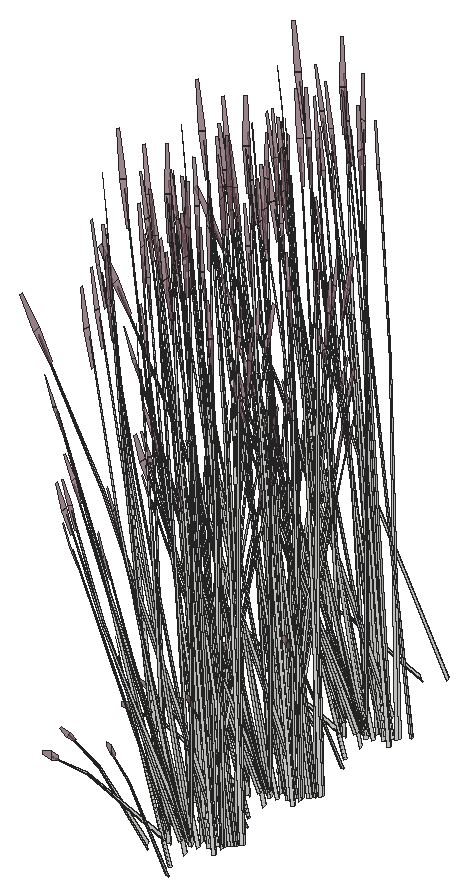
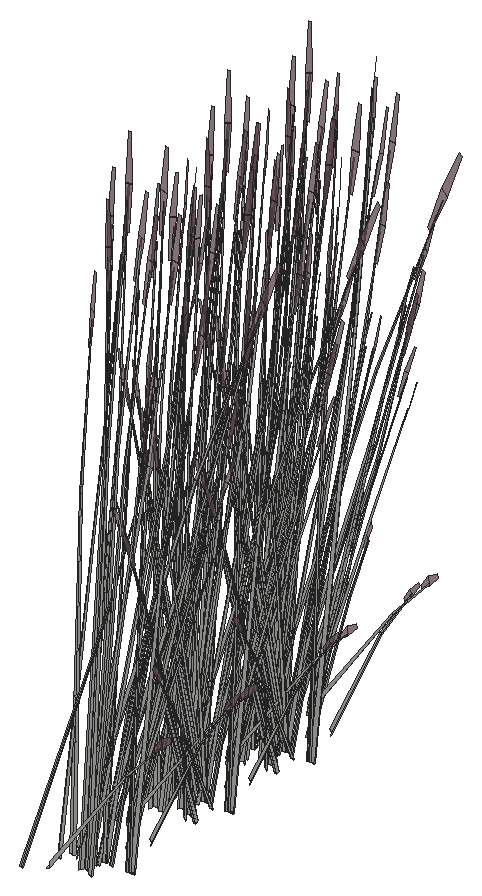
# SketchUp Ruby script. Lengths in inches.
U = 1.inch
M = Sketchup.active_model
def pt(a) = Geom::Point3d.new(a.map { |v| v * U })
def face(e, loops, mat)
  f = e.add_face(loops[0].map { |a| pt(a) })
  loops[1..].each { |l| e.add_face(l.map { |a| pt(a) }).erase! }
  f.material = f.back_material = mat if mat
  f
end
# faces: each face lists its corners as indices into pts; further lists are holes
def faces(e, pts, list, mat = nil) = list.each { |f| face(e, (f[0].is_a?(Array) ? f : [f]).map { |l| l.map { |i| pts[i] } }, mat) }
# xy, xz, yz: faces in a plane at the given z, y or x. An outline is a flat list of corners, or four numbers for a rectangle; further outlines are holes
def ring(l) = l.size == 4 ? [[l[0], l[1]], [l[2], l[1]], [l[2], l[3]], [l[0], l[3]]] : l.each_slice(2).to_a
def flat(e, list, mat, &to3) = list.each { |f| face(e, (f[0].is_a?(Array) ? f : [f]).map { |l| ring(l).map { |u, v| to3.(u, v) } }, mat) }
def xy(e, z, list, mat = nil) = flat(e, list, mat) { |x, y| [x, y, z] }
def xz(e, y, list, mat = nil) = flat(e, list, mat) { |x, z| [x, y, z] }
def yz(e, x, list, mat = nil) = flat(e, list, mat) { |y, z| [x, y, z] }
def lines(e, pts, list) = list.each { |a, b| e.add_line(pt(pts[a]), pt(pts[b])) }
# prism: a flat outline (further loops are holes) pulled along v
def prism(e, loops, v, mat = nil)
  f = face(e, loops, mat); d = Geom::Vector3d.new(v.map { |x| x * U })
  f.pushpull(f.normal.samedirection?(d) ? d.length : -d.length)
end
def box(e, o, s, mat = nil) = prism(e, [[o, [o[0] + s[0], o[1], o[2]], [o[0] + s[0], o[1] + s[1], o[2]], [o[0], o[1] + s[1], o[2]]]], [0, 0, s[2]], mat)
def at(x, y, z, deg = 0) = Geom::Transformation.translation(pt([x, y, z])) * Geom::Transformation.rotation(ORIGIN, Z_AXIS, deg.degrees)
def axes(o, x, y, z) = Geom::Transformation.new([*x, 0, *y, 0, *z, 0, *pt(o).to_a, 1])
def part(name) = M.definitions.add(name)
# library, detail: a bought-in or finely detailed component or shape, given as its bounding box
def library(name, o, s) = part(name).tap { |d| box(d.entities, o, s) }
def detail(e, o, s) = box(e.add_group.entities, o, s)
def put(e, d, t, mat = nil) = e.add_instance(d, t).tap { |i| i.material = mat if mat }
def group(e, t, mat = nil) = e.add_group.tap { |g| g.transformation = t; g.material = mat if mat }.entities
root = M.entities
M.materials.add("LightPink_Translucent").color = [144, 107, 117]
M.materials["LightPink_Translucent"].alpha = 0.75
c1 = part("blade")
p = [[2.15,0.21,22],[0,0.17,0],[0.09,0.45,0],[2.18,0.31,22],[2.29,0.31,22],[0.38,0.45,0],
  [2.48,0.24,33],[2.49,0.24,33],[2.48,0.22,33]]
faces(c1.entities,p,[[0,1,2,3],[4,5,2,3],[6,3,4,7],[8,0,3,6]])
c2 = part("seeds")
p = [[0.3,-0.1,1.38],[-0.01,-0.03,1.59],[-0.01,-0.03,0.03],[0.14,-0.07,-0.07],[0.29,-0.03,3],[0.15,0.01,3.11]]
faces(c2.entities,p,[[0,1,2,3],[1,0,4,5]],"LightPink_Translucent")
c3 = part("blade with seeds")
put(c3.entities,c1,at(0,0,0))
put(c3.entities,c2,axes([2.4,0.25,30.99],[1.5799,-0.05474,1.17369],[-0.12525,1.92788,0.29478],[-0.07173,-0.02425,1.56792]))
put(root,c3,axes([343.98,57.74,7.01],[-0.13683,-0.09148,1.74944],[-0.91315,0.058,-0.27667],[-0.14574,-0.2188,0.14031]))
put(root,c3,axes([344.94,59.28,7.27],[-0.42698,-0.53052,-0.71045],[0.87893,-0.29566,0.08574],[-0.09984,-0.25633,1.00501]))
put(root,c3,axes([344.2,58.1,3.79],[-0.15005,0.02351,1.76342],[-0.82981,-0.26461,-0.26939],[0.01392,-0.22072,0.30037]))
put(root,c3,axes([345.02,58.83,6.82],[0.2697,-0.50175,-0.35414],[0.78684,0.14635,0.4572],[-0.07215,-0.20201,0.87481]))
put(root,c3,axes([344.62,59.17,6.97],[-0.87941,-0.16356,-0.51099],[0.30143,-0.56078,-0.3958],[-0.08064,-0.22578,0.97773]))
put(root,c3,axes([342.87,58.82,7.39],[0.99656,-0.1677,0.53763],[0.17295,0.65785,0.4433],[-0.23438,-0.19388,1.11249]))
put(root,c3,axes([345.37,59.15,7.33],[-0.87543,0.30377,-0.1216],[-0.4302,-0.53915,-0.67495],[-0.1155,-0.2272,1.02557]))
put(root,c3,axes([341.89,58.23,5.06],[0.46666,0.22709,1.1486],[-0.67962,0.13651,0.84392],[-0.14541,-0.17452,0.25299]))
put(root,c3,axes([343.09,58.97,7.02],[0.4066,-0.41448,0.0643],[0.57901,0.24131,0.50621],[-0.18719,-0.13288,0.77189]))
put(root,c3,axes([342.97,61.27,4.39],[-0.36739,-0.66907,-0.69835],[1.05831,-0.24096,-0.18329],[-0.04061,-0.22656,1.54149]))
put(root,c3,axes([345.11,59.36,7.34],[-0.2697,0.50175,0.35414],[-0.78684,-0.14635,-0.4572],[-0.07215,-0.20201,0.87481]))
put(root,c3,axes([344.05,58.5625,4.42],[-0.61821,0.37431,-0.03893],[-0.56645,-0.40995,-0.17649],[-0.03988,-0.11616,0.58215]))
put(root,c3,axes([344.84,63,5.62],[0.77308,0.2631,1.51261],[-0.75736,0.56681,0.59816],[-0.33924,-0.33594,1.26806]))
put(root,c3,axes([343.22,59.44,7.34],[0.13817,0.52554,0.35414],[-0.78985,0.13877,-0.4572],[-0.21215,-0.1506,0.87481]))
put(root,c3,axes([340.8,61.18,4.3125],[0,-0.65246,-0.49651],[1.00089,0,0],[0,-0.1486,1.57504]))
put(root,c3,axes([341.23,61.19,4.32],[0.62448,-0.40708,-0.30978],[0.62448,0.40708,0.30978],[0,-0.13112,1.38974]))
put(root,c3,axes([343.42,61.94,4.96],[-1.00749,-0.31132,-0.29095],[0.48511,-0.65709,-0.50002],[-0.03166,-0.16133,1.59708]))
put(root,c3,axes([341.42,61.48,4.625],[-0.83213,0.54855,0.30756],[-0.83263,-0.54278,-0.36492],[-0.02906,-0.15578,1.64885]))
put(root,c3,axes([343.67,62.625,4.73],[0.23711,-0.77313,-0.23429],[1.12425,0.13477,0.51271],[-0.19645,-0.10677,1.5644]))
put(root,c3,axes([341.23,61.79,4.77],[0,0.65246,0.49651],[-1.00089,0,0],[0,-0.1486,1.57504]))
put(root,c3,axes([343.59,62.3125,4.5],[-0.53742,-0.54764,-0.44739],[0.81403,-0.38564,0.21531],[-0.17391,-0.06776,1.43643]))
put(root,c3,axes([343.7,61.54,4.65],[0.38895,0.72959,0.45755],[-1.11135,0.2537,0.17955],[0.01358,-0.13406,1.58856]))
put(root,c3,axes([343.51,62.11,5.01],[-0.43405,0.58792,0.44739],[-0.90188,-0.28295,-0.21531],[0,-0.13553,1.43643]))
put(root,c3,axes([345.38,62.1875,4.59],[-0.83213,-0.56158,-0.06131],[0.83263,-0.56193,0],[-0.02906,-0.01961,1.75571]))
put(root,c3,axes([343.8,62.25,4.65],[1.13071,0.13747,0.45755],[-0.23011,0.77639,0.17955],[-0.16524,-0.07497,1.58856]))
put(root,c3,axes([343.19,63.49,4.77],[0.96132,-0.17317,0.17642],[0.23737,0.64447,0.35086],[-0.08574,-0.0939,1.60407]))
put(root,c3,axes([344.08,62.81,4.91],[-0.17258,0.58229,0.1448],[-0.84319,-0.10108,-0.41347],[-0.15345,-0.05979,1.26744]))
put(root,c3,axes([346.05,63.53,4.77],[0.25843,-0.64844,0.17642],[0.9457,0.1835,0.35086],[-0.16336,0.00316,1.60407]))
put(root,c3,axes([344.43,63.6,4.49],[-0.90188,-0.29293,0],[0.43405,-0.60866,0],[0,0,1.62707]))
put(root,c3,axes([345.18,62.82,4.76],[-0.87356,-0.52515,-0.25192],[0.73507,-0.5897,0.5513],[-0.23523,0.06143,1.68216]))
put(root,c3,axes([342.88,63.82,4.77],[0.83726,0.32623,0.49651],[-0.50045,0.58498,0],[-0.19069,-0.0743,1.57504]))
put(root,c3,axes([343.98,67.5625,7.01],[-0.13683,-0.09148,1.74944],[-0.91315,0.058,-0.27667],[-0.14574,-0.2188,0.14031]))
put(root,c3,axes([344.94,69.11,7.27],[-0.42698,-0.53052,-0.71045],[0.87893,-0.29566,0.08574],[-0.09984,-0.25633,1.00501]))
put(root,c3,axes([345.6,62.38,5.01],[0.97146,-0.04028,0.44739],[0.08785,0.66859,-0.21531],[-0.17391,0.06776,1.43643]))
put(root,c3,axes([344.74,62.71,4.5],[-0.97146,0.04028,-0.44739],[-0.08785,-0.66859,0.21531],[-0.17391,0.06776,1.43643]))
put(root,c3,axes([344.2,67.93,3.79],[-0.15005,0.02351,1.76342],[-0.82981,-0.26461,-0.26939],[0.01392,-0.22072,0.30037]))
put(root,c3,axes([345.02,68.66,6.82],[0.2697,-0.50175,-0.35414],[0.78684,0.14635,0.4572],[-0.07215,-0.20201,0.87481]))
put(root,c3,axes([345.8125,64.26,4.49],[-0.55235,-0.65609,-0.05142],[0.93577,-0.36461,0.51607],[-0.23059,0.06247,1.6363]))
put(root,c3,axes([345.62,62.67,4.91],[0.66093,0.39201,0.1448],[-0.5513,0.44227,-0.41347],[-0.15345,0.05979,1.26744]))
put(root,c3,axes([344.62,69,6.97],[-0.87941,-0.16356,-0.51099],[0.30143,-0.56078,-0.3958],[-0.08064,-0.22578,0.97773]))
put(root,c3,axes([346.32,63.88,4.77],[0.83726,-0.32623,0.49651],[0.50045,0.58498,0],[-0.19069,0.0743,1.57504]))
put(root,c3,axes([345.5625,64.17,4.32],[-0.83462,-0.16144,-0.30978],[0.21015,-0.56852,0.30978],[-0.16826,0.06556,1.38974]))
put(root,c3,axes([342.87,68.65,7.39],[0.99656,-0.1677,0.53763],[0.17295,0.65785,0.4433],[-0.23438,-0.19388,1.11249]))
put(root,c3,axes([345.37,68.97,7.33],[-0.87543,0.30377,-0.1216],[-0.4302,-0.53915,-0.67495],[-0.1155,-0.2272,1.02557]))
put(root,c3,axes([341.89,68.05,5.06],[0.46666,0.22709,1.1486],[-0.67962,0.13651,0.84392],[-0.14541,-0.17452,0.25299]))
put(root,c3,axes([345.42,62.52,4.96],[0.10425,0.7445,-0.29095],[-1.08575,0.04502,-0.50002],[-0.19119,0.09917,1.59708]))
put(root,c3,axes([343.09,68.79,7.02],[0.4066,-0.41448,0.0643],[0.57901,0.24131,0.50621],[-0.18719,-0.13288,0.77189]))
put(root,c3,axes([344.77,63.09,4.35],[-0.60257,0.49041,-0.62353],[-0.74854,-0.44469,-0.16365],[-0.24146,0.12234,1.37633]))
put(root,c3,axes([342.97,71.1,4.39],[-0.36739,-0.66907,-0.69835],[1.05831,-0.24096,-0.18329],[-0.04061,-0.22656,1.54149]))
put(root,c3,axes([345.84,63.92,4.625],[1.11998,0.21207,0.30756],[-0.2802,0.75803,-0.36492],[-0.18537,0.09487,1.64885]))
put(root,c3,axes([345.76,64.43,4.3125],[-0.83726,0.32623,-0.49651],[-0.50045,-0.58498,0],[-0.19069,0.0743,1.57504]))
put(root,c3,axes([345.11,69.1875,7.34],[-0.2697,0.50175,0.35414],[-0.78684,-0.14635,-0.4572],[-0.07215,-0.20201,0.87481]))
put(root,c3,axes([344.05,68.39,4.42],[-0.61821,0.37431,-0.03893],[-0.56645,-0.40995,-0.17649],[-0.03988,-0.11616,0.58215]))
put(root,c3,axes([341.98,63.63,7.34],[0.60531,-0.34352,0.35414],[0.573,0.39225,-0.4572],[-0.08718,0.19929,0.87481]))
put(root,c3,axes([346.52,64.33,4.67],[0.55932,0.6538,0],[-0.93577,0.36461,-0.51607],[-0.21313,0.08304,1.63711]))
put(root,c3,axes([346.04,61.74,5.13],[-0.02444,-0.61432,1.41272],[1.10603,0.15924,0.59816],[-0.26159,0.33615,1.3335]))
put(root,c3,axes([344.84,72.83,5.62],[0.77308,0.2631,1.51261],[-0.75736,0.56681,0.59816],[-0.33924,-0.33594,1.26806]))
put(root,c3,axes([343.22,69.27,7.34],[0.13817,0.52554,0.35414],[-0.78985,0.13877,-0.4572],[-0.21215,-0.1506,0.87481]))
put(root,c3,axes([340.8,71.01,4.3125],[0,-0.65246,-0.49651],[1.00089,0,0],[0,-0.1486,1.57504]))
put(root,c3,axes([343.4375,64.65,7.02],[-0.6592,0.22175,0.0643],[-0.32265,-0.40436,0.50621],[0.06366,0.17825,0.77189]))
put(root,c3,axes([341.23,71.02,4.32],[0.62448,-0.40708,-0.30978],[0.62448,0.40708,0.30978],[0,-0.13112,1.38974]))
put(root,c3,axes([341.67,64.12,6.82],[-0.60531,0.34352,-0.35414],[-0.573,-0.39225,0.4572],[-0.08718,0.19929,0.87481]))
put(root,c3,axes([341.6,63.73,7.69],[0.98321,0.03233,-0.13498],[-0.02687,0.61208,-0.74919],[-0.0683,0.23574,1.13838]))
put(root,c3,axes([343.67,64.61,7.36],[-0.88151,-0.17057,0.53283],[0.30143,-0.56078,0.43934],[0.05297,0.22053,1.10256]))
put(root,c3,axes([343.42,71.76,4.96],[-1.00749,-0.31132,-0.29095],[0.48511,-0.65709,-0.50002],[-0.03166,-0.16133,1.59708]))
put(root,c3,axes([342.05,65.46,5.06],[-0.02315,-0.38796,1.1486],[0.57853,0.27671,0.84392],[-0.11378,0.18492,0.25299]))
put(root,c3,axes([342.27,63.96,7.3],[0.64041,0.4384,-0.5672],[-0.67652,0.38394,-0.43934],[-0.09744,0.22274,1.08528]))
put(root,c3,axes([341.57,64.62,5.12],[0.8127,-0.11554,0.06507],[0.18684,0.46549,-0.86304],[-0.05152,0.23564,0.7736]))
put(root,c3,axes([341.42,71.31,4.625],[-0.83213,0.54855,0.30756],[-0.83263,-0.54278,-0.36492],[-0.02906,-0.15578,1.64885]))
put(root,c3,axes([342.07,63.76,7.63],[-0.02328,0.60353,-0.7886],[-0.98022,-0.04053,0.09517],[-0.10344,0.25568,1.11556]))
put(root,c3,axes([339.51,65.34,7],[0.10149,-0.03939,1.77383],[0.83886,0.26202,-0.16761],[-0.01971,0.21816,0.31391]))
put(root,c3,axes([343.67,72.45,4.73],[0.23711,-0.77313,-0.23429],[1.12425,0.13477,0.51271],[-0.19645,-0.10677,1.5644]))
put(root,c3,axes([343,63.33,6.17],[-0.0219,-0.25042,1.71376],[0.94901,0.16613,0.13857],[-0.0587,0.35688,0.73262]))
put(root,c3,axes([341.23,71.61,4.77],[0,0.65246,0.49651],[-1.00089,0,0],[0,-0.1486,1.57504]))
put(root,c3,axes([343.59,72.14,4.5],[-0.53742,-0.54764,-0.44739],[0.81403,-0.38564,0.21531],[-0.17391,-0.06776,1.43643]))
put(root,c3,axes([343.7,71.37,4.65],[0.38895,0.72959,0.45755],[-1.11135,0.2537,0.17955],[0.01358,-0.13406,1.58856]))
put(root,c3,axes([343.51,71.94,5.01],[-0.43405,0.58792,0.44739],[-0.90188,-0.28295,-0.21531],[0,-0.13553,1.43643]))
put(root,c3,axes([341.74,64.61,5.66],[0.01966,-0.33682,1.54345],[0.88405,0.17791,0.21329],[-0.0766,0.35897,0.72882]))
put(root,c3,axes([345.38,72.01,4.59],[-0.83213,-0.56158,-0.06131],[0.83263,-0.56193,0],[-0.02906,-0.01961,1.75571]))
put(root,c3,axes([343.8,72.08,4.65],[1.13071,0.13747,0.45755],[-0.23011,0.77639,0.17955],[-0.16524,-0.07497,1.58856]))
put(root,c3,axes([343.19,73.32,4.77],[0.96132,-0.17317,0.17642],[0.23737,0.64447,0.35086],[-0.08574,-0.0939,1.60407]))
put(root,c3,axes([344.08,72.64,4.91],[-0.17258,0.58229,0.1448],[-0.84319,-0.10108,-0.41347],[-0.15345,-0.05979,1.26744]))
put(root,c3,axes([346.05,73.36,4.77],[0.25843,-0.64844,0.17642],[0.9457,0.1835,0.35086],[-0.16336,0.00316,1.60407]))
put(root,c3,axes([344.43,73.42,4.49],[-0.90188,-0.29293,0],[0.43405,-0.60866,0],[0,0,1.62707]))
put(root,c3,axes([345.18,72.64,4.76],[-0.87356,-0.52515,-0.25192],[0.73507,-0.5897,0.5513],[-0.23523,0.06143,1.68216]))
put(root,c3,axes([342.88,73.65,4.77],[0.83726,0.32623,0.49651],[-0.50045,0.58498,0],[-0.19069,-0.0743,1.57504]))
put(root,c3,axes([345.6,72.21,5.01],[0.97146,-0.04028,0.44739],[0.08785,0.66859,-0.21531],[-0.17391,0.06776,1.43643]))
put(root,c3,axes([344.74,72.53,4.5],[-0.97146,0.04028,-0.44739],[-0.08785,-0.66859,0.21531],[-0.17391,0.06776,1.43643]))
put(root,c3,axes([345.8125,74.08,4.49],[-0.55235,-0.65609,-0.05142],[0.93577,-0.36461,0.51607],[-0.23059,0.06247,1.6363]))
put(root,c3,axes([345.62,72.5,4.91],[0.66093,0.39201,0.1448],[-0.5513,0.44227,-0.41347],[-0.15345,0.05979,1.26744]))
put(root,c3,axes([346.32,73.7,4.77],[0.83726,-0.32623,0.49651],[0.50045,0.58498,0],[-0.19069,0.0743,1.57504]))
put(root,c3,axes([345.5625,74,4.32],[-0.83462,-0.16144,-0.30978],[0.21015,-0.56852,0.30978],[-0.16826,0.06556,1.38974]))
put(root,c3,axes([345.42,72.35,4.96],[0.10425,0.7445,-0.29095],[-1.08575,0.04502,-0.50002],[-0.19119,0.09917,1.59708]))
put(root,c3,axes([343.98,79.5625,7.01],[-0.13683,-0.09148,1.74944],[-0.91315,0.058,-0.27667],[-0.14574,-0.2188,0.14031]))
put(root,c3,axes([344.94,81.11,7.27],[-0.42698,-0.53052,-0.71045],[0.87893,-0.29566,0.08574],[-0.09984,-0.25633,1.00501]))
put(root,c3,axes([344.77,72.92,4.35],[-0.60257,0.49041,-0.62353],[-0.74854,-0.44469,-0.16365],[-0.24146,0.12234,1.37633]))
put(root,c3,axes([344.2,79.93,3.79],[-0.15005,0.02351,1.76342],[-0.82981,-0.26461,-0.26939],[0.01392,-0.22072,0.30037]))
put(root,c3,axes([345.84,73.75,4.625],[1.11998,0.21207,0.30756],[-0.2802,0.75803,-0.36492],[-0.18537,0.09487,1.64885]))
put(root,c3,axes([345.76,74.26,4.3125],[-0.83726,0.32623,-0.49651],[-0.50045,-0.58498,0],[-0.19069,0.0743,1.57504]))
put(root,c3,axes([345.02,80.66,6.82],[0.2697,-0.50175,-0.35414],[0.78684,0.14635,0.4572],[-0.07215,-0.20201,0.87481]))
put(root,c3,axes([344.62,81,6.97],[-0.87941,-0.16356,-0.51099],[0.30143,-0.56078,-0.3958],[-0.08064,-0.22578,0.97773]))
put(root,c3,axes([341.98,73.46,7.34],[0.60531,-0.34352,0.35414],[0.573,0.39225,-0.4572],[-0.08718,0.19929,0.87481]))
put(root,c3,axes([346.52,74.16,4.67],[0.55932,0.6538,0],[-0.93577,0.36461,-0.51607],[-0.21313,0.08304,1.63711]))
put(root,c3,axes([346.04,71.57,5.13],[-0.02444,-0.61432,1.41272],[1.10603,0.15924,0.59816],[-0.26159,0.33615,1.3335]))
put(root,c3,axes([342.87,80.65,7.39],[0.99656,-0.1677,0.53763],[0.17295,0.65785,0.4433],[-0.23438,-0.19388,1.11249]))
put(root,c3,axes([345.37,80.97,7.33],[-0.87543,0.30377,-0.1216],[-0.4302,-0.53915,-0.67495],[-0.1155,-0.2272,1.02557]))
put(root,c3,axes([341.89,80.05,5.06],[0.46666,0.22709,1.1486],[-0.67962,0.13651,0.84392],[-0.14541,-0.17452,0.25299]))
put(root,c3,axes([343.09,80.79,7.02],[0.4066,-0.41448,0.0643],[0.57901,0.24131,0.50621],[-0.18719,-0.13288,0.77189]))
put(root,c3,axes([343.4375,74.48,7.02],[-0.6592,0.22175,0.0643],[-0.32265,-0.40436,0.50621],[0.06366,0.17825,0.77189]))
put(root,c3,axes([341.67,73.95,6.82],[-0.60531,0.34352,-0.35414],[-0.573,-0.39225,0.4572],[-0.08718,0.19929,0.87481]))
put(root,c3,axes([342.97,83.1,4.39],[-0.36739,-0.66907,-0.69835],[1.05831,-0.24096,-0.18329],[-0.04061,-0.22656,1.54149]))
put(root,c3,axes([341.6,73.56,7.69],[0.98321,0.03233,-0.13498],[-0.02687,0.61208,-0.74919],[-0.0683,0.23574,1.13838]))
put(root,c3,axes([343.67,74.4375,7.36],[-0.88151,-0.17057,0.53283],[0.30143,-0.56078,0.43934],[0.05297,0.22053,1.10256]))
put(root,c3,axes([342.05,75.28,5.06],[-0.02315,-0.38796,1.1486],[0.57853,0.27671,0.84392],[-0.11378,0.18492,0.25299]))
put(root,c3,axes([345.11,81.1875,7.34],[-0.2697,0.50175,0.35414],[-0.78684,-0.14635,-0.4572],[-0.07215,-0.20201,0.87481]))
put(root,c3,axes([342.27,73.79,7.3],[0.64041,0.4384,-0.5672],[-0.67652,0.38394,-0.43934],[-0.09744,0.22274,1.08528]))
put(root,c3,axes([341.57,74.44,5.12],[0.8127,-0.11554,0.06507],[0.18684,0.46549,-0.86304],[-0.05152,0.23564,0.7736]))
put(root,c3,axes([344.05,80.39,4.42],[-0.61821,0.37431,-0.03893],[-0.56645,-0.40995,-0.17649],[-0.03988,-0.11616,0.58215]))
put(root,c3,axes([342.07,73.59,7.63],[-0.02328,0.60353,-0.7886],[-0.98022,-0.04053,0.09517],[-0.10344,0.25568,1.11556]))
put(root,c3,axes([339.51,75.17,7],[0.10149,-0.03939,1.77383],[0.83886,0.26202,-0.16761],[-0.01971,0.21816,0.31391]))
put(root,c3,axes([344.84,84.83,5.62],[0.77308,0.2631,1.51261],[-0.75736,0.56681,0.59816],[-0.33924,-0.33594,1.26806]))
put(root,c3,axes([343,73.16,6.17],[-0.0219,-0.25042,1.71376],[0.94901,0.16613,0.13857],[-0.0587,0.35688,0.73262]))
put(root,c3,axes([343.22,81.27,7.34],[0.13817,0.52554,0.35414],[-0.78985,0.13877,-0.4572],[-0.21215,-0.1506,0.87481]))
put(root,c3,axes([340.8,83.01,4.3125],[0,-0.65246,-0.49651],[1.00089,0,0],[0,-0.1486,1.57504]))
put(root,c3,axes([341.23,83.02,4.32],[0.62448,-0.40708,-0.30978],[0.62448,0.40708,0.30978],[0,-0.13112,1.38974]))
put(root,c3,axes([343.42,83.76,4.96],[-1.00749,-0.31132,-0.29095],[0.48511,-0.65709,-0.50002],[-0.03166,-0.16133,1.59708]))
put(root,c3,axes([341.74,74.44,5.66],[0.01966,-0.33682,1.54345],[0.88405,0.17791,0.21329],[-0.0766,0.35897,0.72882]))
put(root,c3,axes([341.42,83.31,4.625],[-0.83213,0.54855,0.30756],[-0.83263,-0.54278,-0.36492],[-0.02906,-0.15578,1.64885]))
put(root,c3,axes([343.67,84.45,4.73],[0.23711,-0.77313,-0.23429],[1.12425,0.13477,0.51271],[-0.19645,-0.10677,1.5644]))
put(root,c3,axes([341.23,83.61,4.77],[0,0.65246,0.49651],[-1.00089,0,0],[0,-0.1486,1.57504]))
put(root,c3,axes([343.59,84.14,4.5],[-0.53742,-0.54764,-0.44739],[0.81403,-0.38564,0.21531],[-0.17391,-0.06776,1.43643]))
put(root,c3,axes([343.7,83.37,4.65],[0.38895,0.72959,0.45755],[-1.11135,0.2537,0.17955],[0.01358,-0.13406,1.58856]))
put(root,c3,axes([343.51,83.94,5.01],[-0.43405,0.58792,0.44739],[-0.90188,-0.28295,-0.21531],[0,-0.13553,1.43643]))
put(root,c3,axes([345.38,84.01,4.59],[-0.83213,-0.56158,-0.06131],[0.83263,-0.56193,0],[-0.02906,-0.01961,1.75571]))
put(root,c3,axes([343.8,84.08,4.65],[1.13071,0.13747,0.45755],[-0.23011,0.77639,0.17955],[-0.16524,-0.07497,1.58856]))
put(root,c3,axes([343.19,85.32,4.77],[0.96132,-0.17317,0.17642],[0.23737,0.64447,0.35086],[-0.08574,-0.0939,1.60407]))
put(root,c3,axes([344.08,84.64,4.91],[-0.17258,0.58229,0.1448],[-0.84319,-0.10108,-0.41347],[-0.15345,-0.05979,1.26744]))
put(root,c3,axes([346.05,85.36,4.77],[0.25843,-0.64844,0.17642],[0.9457,0.1835,0.35086],[-0.16336,0.00316,1.60407]))
put(root,c3,axes([344.43,85.42,4.49],[-0.90188,-0.29293,0],[0.43405,-0.60866,0],[0,0,1.62707]))
put(root,c3,axes([345.18,84.64,4.76],[-0.87356,-0.52515,-0.25192],[0.73507,-0.5897,0.5513],[-0.23523,0.06143,1.68216]))
put(root,c3,axes([342.88,85.65,4.77],[0.83726,0.32623,0.49651],[-0.50045,0.58498,0],[-0.19069,-0.0743,1.57504]))
put(root,c3,axes([345.6,84.21,5.01],[0.97146,-0.04028,0.44739],[0.08785,0.66859,-0.21531],[-0.17391,0.06776,1.43643]))
put(root,c3,axes([344.74,84.53,4.5],[-0.97146,0.04028,-0.44739],[-0.08785,-0.66859,0.21531],[-0.17391,0.06776,1.43643]))
put(root,c3,axes([343.98,90.03,7.01],[-0.13683,-0.09148,1.74944],[-0.91315,0.058,-0.27667],[-0.14574,-0.2188,0.14031]))
put(root,c3,axes([344.94,91.58,7.27],[-0.42698,-0.53052,-0.71045],[0.87893,-0.29566,0.08574],[-0.09984,-0.25633,1.00501]))
